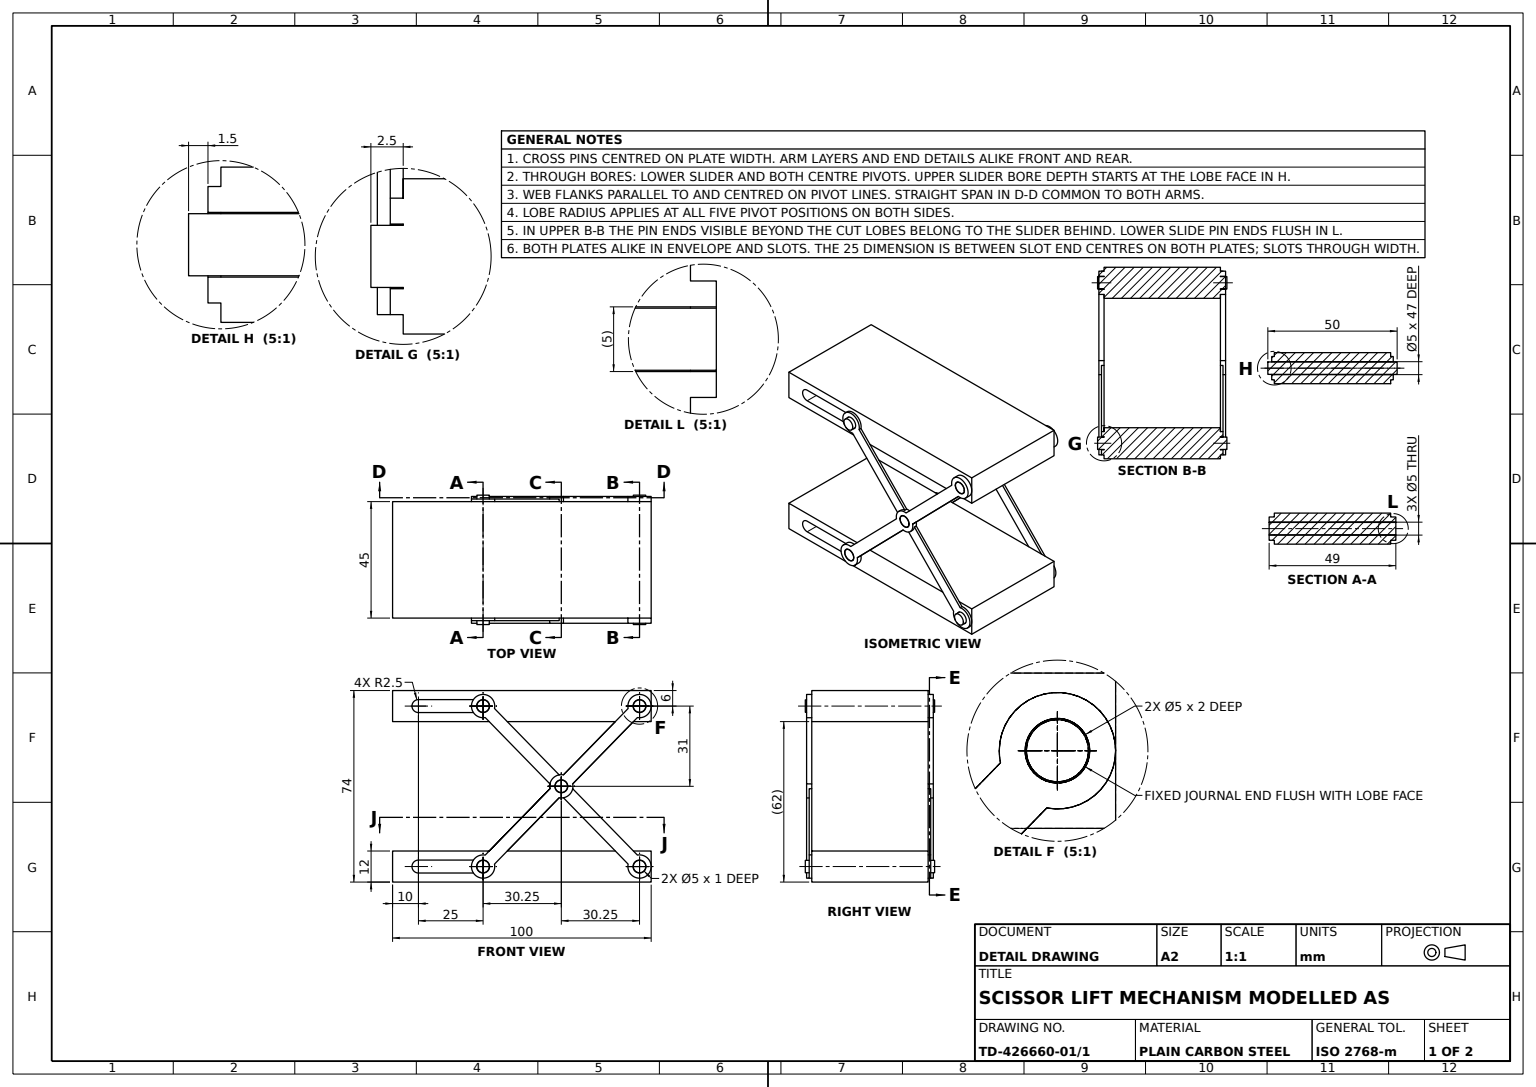
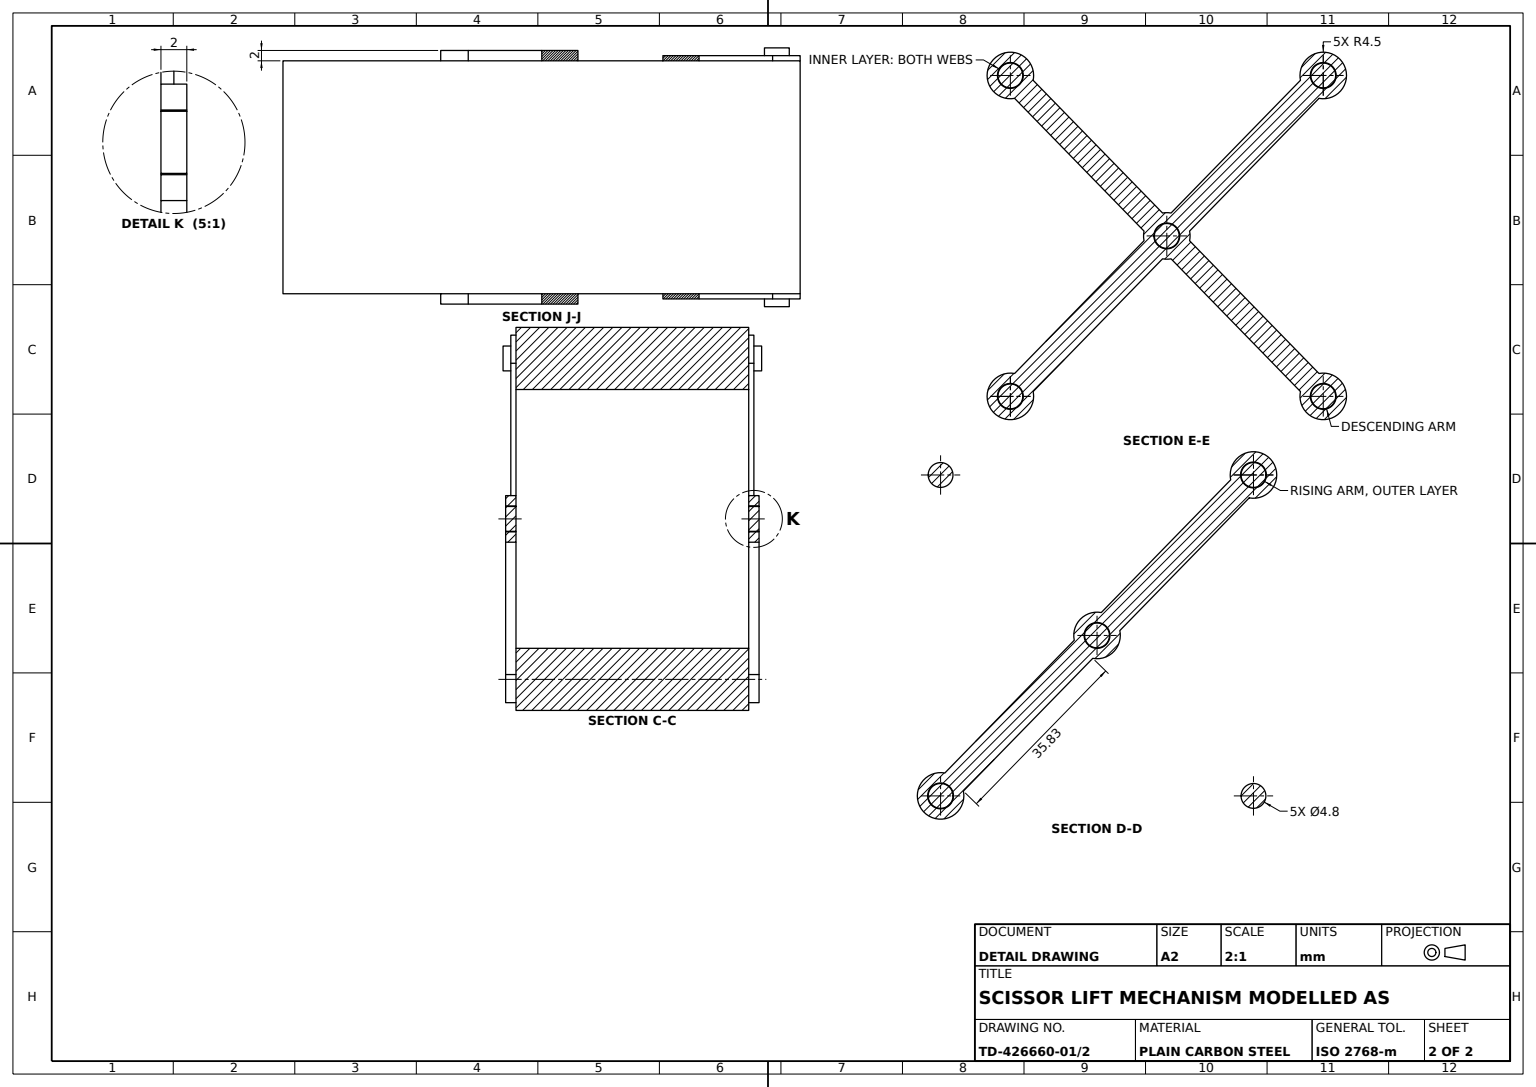
solid
v1 (-17.4,68,-25)
v2 (-12.6,68,-25)
e1 v1 v2 CIRCLE(AX(P(-15,68,-25),D(0,0,-1),D(-1,0,0)),2.4)
e2 v2 v1 CIRCLE(AX(P(-15,68,-25),D(0,0,-1),D(-1,0,0)),2.4)
face PLANE(AX(P(-15,68,-25),D(0,0,-1),D(-1,0,0))) [e1 e2]
v3 (-12.6,68,25)
e3 v3 v2 LINE
v4 (-17.4,68,25)
e4 v4 v3 CIRCLE(AX(P(-15,68,25),D(0,0,1),D(1,0,0)),2.4)
e5 v4 v1 LINE
face CYL(AX(P(-15,68,25),D(0,0,-1),D(-1,0,0)),2.4) [-e3 -e4 e5 -e2]
e6 v3 v4 CIRCLE(AX(P(-15,68,25),D(0,0,1),D(1,0,0)),2.4)
face PLANE(AX(P(-15,68,25),D(0,0,1),D(1,0,0))) [e4 e6]
face CYL(AX(P(-15,68,25),D(0,0,-1),D(-1,0,0)),2.4) [-e5 -e6 e3 -e1]
solid
v5 (17.65,37,22.5)
v6 (12.85,37,22.5)
e7 v5 v6 CIRCLE(AX(P(15.25,37,22.5),D(0,0,1),D(1,0,0)),2.4)
e8 v6 v5 CIRCLE(AX(P(15.25,37,22.5),D(0,0,1),D(1,0,0)),2.4)
face PLANE(AX(P(15.25,37,22.5),D(0,0,1),D(1,0,0))) rev [-e7 -e8]
v7 (17.65,37,24.5)
v8 (12.85,37,24.5)
e9 v7 v8 CIRCLE(AX(P(15.25,37,24.5),D(0,0,1),D(1,0,0)),2.4)
e10 v8 v7 CIRCLE(AX(P(15.25,37,24.5),D(0,0,1),D(1,0,0)),2.4)
face PLANE(AX(P(15.25,37,24.5),D(0,0,1),D(1,0,0))) [e9 e10]
e11 v5 v7 LINE
e12 v6 v8 LINE
face CYL(AX(P(15.25,37,22.5),D(0,0,1),D(1,0,0)),2.4) [-e9 -e11 e7 e12]
face CYL(AX(P(15.25,37,22.5),D(0,0,1),D(1,0,0)),2.4) [e11 -e10 -e12 e8]
solid
v9 (12.85,37,-22.5)
v10 (12.85,37,-24.5)
e13 v9 v10 LINE
v11 (17.65,37,-24.5)
e14 v11 v10 CIRCLE(AX(P(15.25,37,-24.5),D(0,0,-1),D(-1,0,0)),2.4)
v12 (17.65,37,-22.5)
e15 v12 v11 LINE
e16 v12 v9 CIRCLE(AX(P(15.25,37,-22.5),D(0,0,-1),D(-1,0,0)),2.4)
face CYL(AX(P(15.25,37,-22.5),D(0,0,-1),D(-1,0,0)),2.4) [e13 -e14 -e15 e16]
e17 v10 v11 CIRCLE(AX(P(15.25,37,-24.5),D(0,0,-1),D(-1,0,0)),2.4)
face PLANE(AX(P(15.25,37,-24.5),D(0,0,-1),D(-1,0,0))) [e17 e14]
e18 v9 v12 CIRCLE(AX(P(15.25,37,-22.5),D(0,0,-1),D(-1,0,0)),2.4)
face PLANE(AX(P(15.25,37,-22.5),D(0,0,-1),D(-1,0,0))) rev [-e18 -e16]
face CYL(AX(P(15.25,37,-22.5),D(0,0,-1),D(-1,0,0)),2.4) [e15 -e17 -e13 e18]
solid
v13 (-12.6,6,-24.5)
v14 (-12.6,6,24.5)
e19 v13 v14 LINE
v15 (-17.4,6,24.5)
e20 v15 v14 CIRCLE(AX(P(-15,6,24.5),D(0,0,1),D(1,0,0)),2.4)
v16 (-17.4,6,-24.5)
e21 v16 v15 LINE
e22 v16 v13 CIRCLE(AX(P(-15,6,-24.5),D(0,0,1),D(1,0,0)),2.4)
face CYL(AX(P(-15,6,-24.5),D(0,0,1),D(1,0,0)),2.4) [e19 -e20 -e21 e22]
e23 v14 v15 CIRCLE(AX(P(-15,6,24.5),D(0,0,1),D(1,0,0)),2.4)
face PLANE(AX(P(-15,6,24.5),D(0,0,1),D(1,0,0))) [e23 e20]
e24 v13 v16 CIRCLE(AX(P(-15,6,-24.5),D(0,0,1),D(1,0,0)),2.4)
face PLANE(AX(P(-15,6,-24.5),D(0,0,1),D(1,0,0))) rev [-e22 -e24]
face CYL(AX(P(-15,6,-24.5),D(0,0,1),D(1,0,0)),2.4) [e21 -e23 -e19 e24]
solid
v17 (12.75,37,24.5)
v18 (17.75,37,24.5)
e25 v17 v18 CIRCLE(AX(P(15.25,37,24.5),D(0,0,1),D(1,0,0)),2.5)
v19 (17.75,37,22.5)
e26 v18 v19 LINE
v20 (12.75,37,22.5)
e27 v20 v19 CIRCLE(AX(P(15.25,37,22.5),D(0,0,1),D(1,0,0)),2.5)
e28 v17 v20 LINE
face CYL(AX(P(15.25,37,23.5),D(0,0,-1),D(-1,0,0)),2.5) rev [e25 e26 -e27 -e28]
v21 (47.9,68,-22.5)
v22 (43.1,68,-22.5)
e29 v21 v22 CIRCLE(AX(P(45.5,68,-22.5),D(0,0,-1),D(1,0,0)),2.4)
v23 (43.1,68,-24.5)
e30 v23 v22 LINE
v24 (47.9,68,-24.5)
e31 v24 v23 CIRCLE(AX(P(45.5,68,-24.5),D(0,0,-1),D(-1,0,0)),2.4)
e32 v24 v21 LINE
face CYL(AX(P(45.5,68,-24.5),D(0,0,1),D(1,0,0)),2.4) [e29 -e30 -e31 e32]
v25 (-40,8.5,22.5)
v26 (-40,3.5,22.5)
e33 v25 v26 CIRCLE(AX(P(-40,6,22.5),D(0,0,1),D(1,0,0)),2.5)
v27 (-40,3.5,-22.5)
e34 v27 v26 LINE
v28 (-40,8.5,-22.5)
e35 v28 v27 CIRCLE(AX(P(-40,6,-22.5),D(0,0,1),D(1,0,0)),2.5)
e36 v28 v25 LINE
face CYL(AX(P(-40,6,-177.5),D(0,0,1),D(1,0,0)),2.5) rev [e33 -e34 -e35 e36]
v29 (50,68,-22.5)
v30 (44.67612,63.576063,-22.5)
e37 v29 v30 CIRCLE(AX(P(45.5,68,-22.5),D(0,0,-1),D(-1,0,0)),4.5)
v31 (44.67612,63.576063,-24.5)
e38 v31 v30 LINE
v32 (50,68,-24.5)
e39 v32 v31 CIRCLE(AX(P(45.5,68,-24.5),D(0,0,-1),D(-1,0,0)),4.5)
e40 v32 v29 LINE
face CYL(AX(P(45.5,68,-24.5),D(0,0,1),D(1,0,0)),4.5) [e37 -e38 -e39 e40]
v33 (43,6,23.5)
v34 (43,6,22.5)
e41 v33 v34 LINE
v35 (48,6,22.5)
e42 v35 v34 CIRCLE(AX(P(45.5,6,22.5),D(0,0,1),D(1,0,0)),2.5)
v36 (48,6,23.5)
e43 v36 v35 LINE
e44 v36 v33 CIRCLE(AX(P(45.5,6,23.5),D(0,0,1),D(1,0,0)),2.5)
face CYL(AX(P(45.5,6,23.5),D(0,0,-1),D(-1,0,0)),2.5) rev [e41 -e42 -e43 e44]
v37 (-12.638188,12,-22.5)
v38 (10.847563,36.068042,-22.5)
e45 v37 v38 LINE
v39 (10.847563,36.068042,-24.5)
e46 v39 v38 LINE
v40 (-14.17612,10.423937,-24.5)
e47 v40 v39 LINE
v41 (-14.17612,10.423937,-22.5)
e48 v40 v41 LINE
e49 v41 v37 LINE
face PLANE(AX(P(10.847563,36.068042,-24.5),D(0.715711578,-0.698395975,0),D(0.698395975,0.715711578,0))) rev [e45 -e46 -e47 e48 e49]
v42 (16.07388,32.576063,-22.5)
v43 (14.42612,32.576063,-22.5)
e50 v42 v43 CIRCLE(AX(P(15.25,37,-22.5),D(0,0,-1),D(-1,0,0)),4.5)
v44 (14.42612,32.576063,-24.5)
e51 v44 v43 LINE
v45 (19.75,37,-24.5)
e52 v45 v44 CIRCLE(AX(P(15.25,37,-24.5),D(0,0,-1),D(-1,0,0)),4.5)
v46 (19.75,37,-22.5)
e53 v45 v46 LINE
v47 (19.652437,36.068042,-22.5)
e54 v46 v47 CIRCLE(AX(P(15.25,37,-22.5),D(0,0,-1),D(-1,0,0)),4.5)
v48 (19.652437,36.068042,-23.5)
e55 v48 v47 LINE
v49 (16.07388,32.576063,-23.5)
e56 v49 v48 CIRCLE(AX(P(15.25,37,-23.5),D(0,0,1),D(-1,0,0)),4.5)
e57 v49 v42 LINE
face CYL(AX(P(15.25,37,-23.5),D(0,0,1),D(1,0,0)),4.5) [e50 -e51 -e52 e53 e54 -e55 -e56 e57]
v50 (-19.5,6,-24.5)
e58 v50 v40 CIRCLE(AX(P(-15,6,-24.5),D(0,0,-1),D(-1,0,0)),4.5)
v51 (-19.5,6,-22.5)
e59 v50 v51 LINE
v52 (-18.741657,8.5,-22.5)
e60 v51 v52 CIRCLE(AX(P(-15,6,-22.5),D(0,0,-1),D(-1,0,0)),4.5)
e61 v52 v41 CIRCLE(AX(P(-15,6,-22.5),D(0,0,-1),D(-1,0,0)),4.5)
face CYL(AX(P(-15,6,-24.5),D(0,0,1),D(1,0,0)),4.5) [-e58 e59 e60 e61 -e48]
v53 (41,6,-23.5)
v54 (41.097563,6.931958,-23.5)
e62 v53 v54 CIRCLE(AX(P(45.5,6,-23.5),D(0,0,-1),D(-1,0,0)),4.5)
v55 (41,6,-22.5)
e63 v53 v55 LINE
v56 (41.097563,6.931958,-22.5)
e64 v55 v56 CIRCLE(AX(P(45.5,6,-22.5),D(0,0,-1),D(-1,0,0)),4.5)
e65 v54 v56 LINE
face CYL(AX(P(45.5,6,-23.5),D(0,0,1),D(1,0,0)),4.5) [-e62 e63 e64 -e65]
v57 (41,6,23.5)
v58 (41,6,22.5)
e66 v57 v58 LINE
v59 (41.097563,6.931958,23.5)
e67 v59 v57 CIRCLE(AX(P(45.5,6,23.5),D(0,0,1),D(1,0,0)),4.5)
v60 (41.097563,6.931958,22.5)
e68 v59 v60 LINE
e69 v60 v58 CIRCLE(AX(P(45.5,6,22.5),D(0,0,1),D(1,0,0)),4.5)
face CYL(AX(P(45.5,6,23.5),D(0,0,-1),D(-1,0,0)),4.5) [-e66 -e67 e68 e69]
v61 (-5.652134,12,-22.5)
v62 (-10.597563,6.931958,-22.5)
e70 v61 v62 LINE
v63 (36.152134,12,-22.5)
e71 v63 v61 LINE
e72 v56 v63 LINE
v64 (50,6,-22.5)
e73 v64 v55 CIRCLE(AX(P(45.5,6,-22.5),D(0,0,-1),D(-1,0,0)),4.5)
v65 (50,0,-22.5)
e74 v64 v65 LINE
v66 (-50,0,-22.5)
e75 v65 v66 LINE
v67 (-50,12,-22.5)
e76 v67 v66 LINE
e77 v37 v67 LINE
e78 v52 v28 LINE
v68 (-18.741657,3.5,-22.5)
e79 v27 v68 LINE
v69 (-10.5,6,-22.5)
e80 v69 v68 CIRCLE(AX(P(-15,6,-22.5),D(0,0,-1),D(-1,0,0)),4.5)
e81 v62 v69 CIRCLE(AX(P(-15,6,-22.5),D(0,0,-1),D(-1,0,0)),4.5)
face PLANE(AX(P(-50,12,-22.5),D(0,0,1),D(1,0,0))) rev [-e70 -e71 -e72 -e64 -e73 e74 e75 -e76 -e77 -e49 -e61 e78 e35 e79 -e80 -e81]
v70 (-15,3.5,-22.5)
v71 (-15,3.5,22.5)
e82 v70 v71 LINE
e83 v68 v70 LINE
v72 (-18.741657,3.5,22.5)
e84 v26 v72 LINE
e85 v71 v72 LINE
face PLANE(AX(P(-15,3.5,-177.5),D(0,-1,0),D(1,0,0))) rev [-e82 -e83 -e79 e34 e84 -e85]
v73 (14.42612,41.423937,23.5)
v74 (14.42612,41.423937,22.5)
e86 v73 v74 LINE
v75 (10.847563,37.931958,23.5)
e87 v75 v73 CIRCLE(AX(P(15.25,37,23.5),D(0,0,-1),D(1,0,0)),4.5)
v76 (10.847563,37.931958,22.5)
e88 v75 v76 LINE
v77 (10.75,37,22.5)
e89 v76 v77 CIRCLE(AX(P(15.25,37,22.5),D(0,0,1),D(1,0,0)),4.5)
v78 (10.75,37,24.5)
e90 v78 v77 LINE
v79 (16.07388,41.423937,24.5)
e91 v79 v78 CIRCLE(AX(P(15.25,37,24.5),D(0,0,1),D(1,0,0)),4.5)
v80 (16.07388,41.423937,22.5)
e92 v79 v80 LINE
e93 v80 v74 CIRCLE(AX(P(15.25,37,22.5),D(0,0,1),D(1,0,0)),4.5)
face CYL(AX(P(15.25,37,23.5),D(0,0,-1),D(-1,0,0)),4.5) [-e86 -e87 e88 e89 -e90 -e91 e92 e93]
v81 (47.9,6,22.5)
v82 (43.1,6,22.5)
e94 v81 v82 CIRCLE(AX(P(45.5,6,22.5),D(0,0,1),D(-1,0,0)),2.4)
v83 (43.1,6,25)
e95 v83 v82 LINE
v84 (47.9,6,25)
e96 v84 v83 CIRCLE(AX(P(45.5,6,25),D(0,0,1),D(1,0,0)),2.4)
e97 v84 v81 LINE
face CYL(AX(P(45.5,6,25),D(0,0,-1),D(-1,0,0)),2.4) [e94 -e95 -e96 e97]
v85 (16.07388,32.576063,23.5)
e98 v85 v59 LINE
v86 (16.07388,32.576063,22.5)
e99 v85 v86 LINE
v87 (36.152134,12,22.5)
e100 v86 v87 LINE
e101 v87 v60 LINE
face PLANE(AX(P(16.07388,32.576063,23.5),D(0.715711578,0.698395975,0),D(-0.698395975,0.715711578,0))) rev [-e68 -e98 e99 e100 e101]
v88 (10.847563,36.068042,22.5)
e102 v77 v88 CIRCLE(AX(P(15.25,37,22.5),D(0,0,1),D(1,0,0)),4.5)
v89 (10.847563,36.068042,24.5)
e103 v89 v88 LINE
e104 v78 v89 CIRCLE(AX(P(15.25,37,24.5),D(0,0,1),D(1,0,0)),4.5)
face CYL(AX(P(15.25,37,23.5),D(0,0,-1),D(-1,0,0)),4.5) [e90 e102 -e103 -e104]
e105 v82 v81 CIRCLE(AX(P(45.5,6,22.5),D(0,0,1),D(-1,0,0)),2.4)
e106 v83 v84 CIRCLE(AX(P(45.5,6,25),D(0,0,1),D(1,0,0)),2.4)
face CYL(AX(P(45.5,6,25),D(0,0,-1),D(-1,0,0)),2.4) [e95 e105 -e97 -e106]
v90 (41,68,-22.5)
e107 v90 v29 CIRCLE(AX(P(45.5,68,-22.5),D(0,0,-1),D(-1,0,0)),4.5)
v91 (41,68,-24.5)
e108 v91 v32 CIRCLE(AX(P(45.5,68,-24.5),D(0,0,-1),D(-1,0,0)),4.5)
e109 v91 v90 LINE
face CYL(AX(P(45.5,68,-24.5),D(0,0,1),D(1,0,0)),4.5) [e107 -e40 -e108 e109]
v92 (47.9,68,24.5)
v93 (47.9,68,22.5)
e110 v92 v93 LINE
v94 (43.1,68,24.5)
e111 v94 v92 CIRCLE(AX(P(45.5,68,24.5),D(0,0,1),D(1,0,0)),2.4)
v95 (43.1,68,22.5)
e112 v94 v95 LINE
e113 v95 v93 CIRCLE(AX(P(45.5,68,22.5),D(0,0,1),D(-1,0,0)),2.4)
face CYL(AX(P(45.5,68,24.5),D(0,0,-1),D(-1,0,0)),2.4) [-e110 -e111 e112 e113]
v96 (-50,62,-22.5)
v97 (-50,62,22.5)
e114 v96 v97 LINE
v98 (-50,74,22.5)
e115 v98 v97 LINE
v99 (-50,74,-22.5)
e116 v99 v98 LINE
e117 v99 v96 LINE
face PLANE(AX(P(-50,74,-22.5),D(1,0,0),D(0,0,-1))) rev [e114 -e115 -e116 e117]
v100 (19.652437,37.931958,-24.5)
e118 v31 v100 LINE
v101 (43.138188,62,-22.5)
e119 v30 v101 LINE
v102 (19.652437,37.931958,-22.5)
e120 v101 v102 LINE
e121 v100 v102 LINE
face PLANE(AX(P(44.67612,63.576063,-24.5),D(-0.715711578,0.698395975,0),D(-0.698395975,-0.715711578,0))) rev [-e118 e38 e119 e120 -e121]
v103 (50,62,-22.5)
e122 v29 v103 LINE
v104 (50,74,-22.5)
e123 v104 v29 LINE
v105 (50,74,22.5)
e124 v105 v104 LINE
v106 (50,68,22.5)
e125 v105 v106 LINE
v107 (50,62,22.5)
e126 v106 v107 LINE
e127 v107 v103 LINE
face PLANE(AX(P(50,74,-22.5),D(-1,0,0),D(0,0,1))) rev [-e122 -e123 -e124 e125 e126 e127]
v108 (14.42612,41.423937,-23.5)
v109 (14.42612,41.423937,-22.5)
e128 v108 v109 LINE
v110 (-10.597563,67.068042,-23.5)
e129 v110 v108 LINE
v111 (-10.597563,67.068042,-22.5)
e130 v110 v111 LINE
v112 (-5.652134,62,-22.5)
e131 v111 v112 LINE
e132 v112 v109 LINE
face PLANE(AX(P(14.42612,41.423937,-23.5),D(-0.715711578,-0.698395975,0),D(0.698395975,-0.715711578,0))) rev [-e128 -e129 e130 e131 e132]
e133 v68 v51 CIRCLE(AX(P(-15,6,-22.5),D(0,0,-1),D(-1,0,0)),4.5)
v113 (-10.5,6,-24.5)
e134 v113 v50 CIRCLE(AX(P(-15,6,-24.5),D(0,0,-1),D(-1,0,0)),4.5)
e135 v113 v69 LINE
face CYL(AX(P(-15,6,-24.5),D(0,0,1),D(1,0,0)),4.5) [e80 e133 -e59 -e134 e135]
v114 (50,12,22.5)
v115 (50,12,-22.5)
e136 v114 v115 LINE
v116 (43.138188,12,-22.5)
e137 v115 v116 LINE
e138 v116 v63 LINE
e139 v61 v37 LINE
v117 (-50,12,22.5)
e140 v67 v117 LINE
v118 (-12.638188,12,22.5)
e141 v117 v118 LINE
v119 (-5.652134,12,22.5)
e142 v118 v119 LINE
e143 v119 v87 LINE
v120 (43.138188,12,22.5)
e144 v87 v120 LINE
e145 v120 v114 LINE
face PLANE(AX(P(0,12,0),D(0,1,0),D(0,0,1))) [e136 e137 e138 e71 e139 e77 e140 e141 e142 e143 e144 e145]
e146 v22 v21 CIRCLE(AX(P(45.5,68,-22.5),D(0,0,-1),D(1,0,0)),2.4)
e147 v23 v24 CIRCLE(AX(P(45.5,68,-24.5),D(0,0,-1),D(-1,0,0)),2.4)
face CYL(AX(P(45.5,68,-24.5),D(0,0,1),D(1,0,0)),2.4) [e146 -e32 -e147 e30]
v121 (10.847563,37.931958,-23.5)
v122 (-14.17612,63.576063,-23.5)
e148 v121 v122 LINE
v123 (10.847563,37.931958,-22.5)
e149 v121 v123 LINE
v124 (-12.638188,62,-22.5)
e150 v123 v124 LINE
v125 (-14.17612,63.576063,-22.5)
e151 v124 v125 LINE
e152 v122 v125 LINE
face PLANE(AX(P(10.847563,37.931958,-23.5),D(0.715711578,0.698395975,0),D(-0.698395975,0.715711578,0))) rev [-e148 e149 e150 e151 -e152]
v126 (-15,8.5,-22.5)
v127 (-15,8.5,22.5)
e153 v126 v127 LINE
v128 (-18.741657,8.5,22.5)
e154 v127 v128 LINE
e155 v128 v25 LINE
e156 v126 v52 LINE
face PLANE(AX(P(-15,8.5,-177.5),D(0,1,0),D(0,0,1))) rev [e153 e154 e155 -e36 -e78 -e156]
v129 (41,68,24.5)
v130 (41,68,22.5)
e157 v129 v130 LINE
v131 (50,68,24.5)
e158 v131 v129 CIRCLE(AX(P(45.5,68,24.5),D(0,0,1),D(1,0,0)),4.5)
e159 v131 v106 LINE
e160 v106 v130 CIRCLE(AX(P(45.5,68,22.5),D(0,0,1),D(1,0,0)),4.5)
face CYL(AX(P(45.5,68,24.5),D(0,0,-1),D(-1,0,0)),4.5) [-e157 -e158 e159 e160]
v132 (44.67612,10.423937,22.5)
e161 v132 v120 LINE
v133 (50,6,22.5)
e162 v133 v132 CIRCLE(AX(P(45.5,6,22.5),D(0,0,1),D(1,0,0)),4.5)
e163 v114 v133 LINE
face PLANE(AX(P(-50,12,22.5),D(0,0,-1),D(-1,0,0))) rev [-e145 -e161 -e162 -e163]
v134 (50,6,23.5)
e164 v134 v133 LINE
e165 v57 v134 CIRCLE(AX(P(45.5,6,23.5),D(0,0,1),D(1,0,0)),4.5)
e166 v58 v133 CIRCLE(AX(P(45.5,6,22.5),D(0,0,1),D(1,0,0)),4.5)
face CYL(AX(P(45.5,6,23.5),D(0,0,-1),D(-1,0,0)),4.5) [-e164 -e165 e66 e166]
e167 v92 v94 CIRCLE(AX(P(45.5,68,24.5),D(0,0,1),D(1,0,0)),2.4)
e168 v93 v95 CIRCLE(AX(P(45.5,68,22.5),D(0,0,1),D(-1,0,0)),2.4)
face CYL(AX(P(45.5,68,24.5),D(0,0,-1),D(-1,0,0)),2.4) [-e112 -e167 e110 e168]
v135 (-10.5,68,-22.5)
e169 v135 v111 CIRCLE(AX(P(-15,68,-22.5),D(0,0,-1),D(-1,0,0)),4.5)
v136 (-18.741657,70.5,-22.5)
e170 v136 v135 CIRCLE(AX(P(-15,68,-22.5),D(0,0,-1),D(-1,0,0)),4.5)
v137 (-40,70.5,-22.5)
e171 v136 v137 LINE
v138 (-40,65.5,-22.5)
e172 v137 v138 CIRCLE(AX(P(-40,68,-22.5),D(0,0,1),D(1,0,0)),2.5)
v139 (-18.741657,65.5,-22.5)
e173 v138 v139 LINE
e174 v125 v139 CIRCLE(AX(P(-15,68,-22.5),D(0,0,-1),D(-1,0,0)),4.5)
e175 v124 v96 LINE
e176 v104 v99 LINE
v140 (41.097563,67.068042,-22.5)
e177 v140 v90 CIRCLE(AX(P(45.5,68,-22.5),D(0,0,-1),D(-1,0,0)),4.5)
v141 (36.152134,62,-22.5)
e178 v141 v140 LINE
e179 v141 v112 LINE
face PLANE(AX(P(-50,74,-22.5),D(0,0,1),D(1,0,0))) rev [-e169 -e170 e171 e172 e173 -e174 -e151 e175 -e117 -e176 e123 -e107 -e177 -e178 e179 -e131]
v142 (44.67612,10.423937,-23.5)
e180 v48 v142 LINE
e181 v47 v116 LINE
v143 (44.67612,10.423937,-22.5)
e182 v116 v143 LINE
e183 v142 v143 LINE
face PLANE(AX(P(44.67612,10.423937,-23.5),D(-0.715711578,-0.698395975,0),D(0.698395975,-0.715711578,0))) rev [-e180 e55 e181 e182 -e183]
v144 (48,68,-22.5)
v145 (43,68,-22.5)
e184 v144 v145 CIRCLE(AX(P(45.5,68,-22.5),D(0,0,-1),D(-1,0,0)),2.5)
e185 v145 v144 CIRCLE(AX(P(45.5,68,-22.5),D(0,0,-1),D(-1,0,0)),2.5)
face PLANE(AX(P(-50,74,-22.5),D(0,0,1),D(1,0,0))) rev [e184 e185] [-e29 -e146]
v146 (47.9,6,-25)
v147 (47.9,6,-22.5)
e186 v146 v147 LINE
v148 (43.1,6,-22.5)
e187 v147 v148 CIRCLE(AX(P(45.5,6,-22.5),D(0,0,-1),D(1,0,0)),2.4)
v149 (43.1,6,-25)
e188 v149 v148 LINE
e189 v146 v149 CIRCLE(AX(P(45.5,6,-25),D(0,0,-1),D(-1,0,0)),2.4)
face CYL(AX(P(45.5,6,-25),D(0,0,1),D(1,0,0)),2.4) [e186 e187 -e188 -e189]
v150 (48,6,-23.5)
v151 (48,6,-22.5)
e190 v150 v151 LINE
v152 (43,6,-23.5)
e191 v150 v152 CIRCLE(AX(P(45.5,6,-23.5),D(0,0,-1),D(-1,0,0)),2.5)
v153 (43,6,-22.5)
e192 v152 v153 LINE
e193 v151 v153 CIRCLE(AX(P(45.5,6,-22.5),D(0,0,-1),D(-1,0,0)),2.5)
face CYL(AX(P(45.5,6,-23.5),D(0,0,1),D(1,0,0)),2.5) rev [-e190 e191 e192 -e193]
e194 v98 v105 LINE
face PLANE(AX(P(0,74,0),D(0,1,0),D(0,0,1))) [e194 e124 e176 e116]
v154 (43.138188,62,22.5)
v155 (44.67612,63.576063,22.5)
e195 v154 v155 LINE
v156 (44.67612,63.576063,24.5)
e196 v156 v155 LINE
v157 (19.652437,37.931958,24.5)
e197 v157 v156 LINE
v158 (19.652437,37.931958,22.5)
e198 v157 v158 LINE
e199 v158 v154 LINE
face PLANE(AX(P(19.652437,37.931958,24.5),D(-0.715711578,0.698395975,0),D(-0.698395975,-0.715711578,0))) rev [e195 -e196 -e197 e198 e199]
v159 (-10.5,68,-23.5)
e200 v159 v110 CIRCLE(AX(P(-15,68,-23.5),D(0,0,-1),D(-1,0,0)),4.5)
e201 v159 v135 LINE
face CYL(AX(P(-15,68,-23.5),D(0,0,1),D(1,0,0)),4.5) [-e130 -e200 e201 e169]
v160 (14.42612,32.576063,24.5)
v161 (14.42612,32.576063,22.5)
e202 v160 v161 LINE
v162 (-10.597563,6.931958,24.5)
e203 v162 v160 LINE
v163 (-10.597563,6.931958,22.5)
e204 v162 v163 LINE
e205 v163 v119 LINE
e206 v119 v161 LINE
face PLANE(AX(P(-10.597563,6.931958,24.5),D(-0.715711578,0.698395975,0),D(-0.698395975,-0.715711578,0))) rev [-e202 -e203 e204 e205 e206]
v164 (-15,65.5,-22.5)
v165 (-15,65.5,22.5)
e207 v164 v165 LINE
e208 v139 v164 LINE
v166 (-40,65.5,22.5)
e209 v138 v166 LINE
v167 (-18.741657,65.5,22.5)
e210 v166 v167 LINE
e211 v167 v165 LINE
face PLANE(AX(P(-15,65.5,-27.5),D(0,-1,0),D(1,0,0))) rev [-e207 -e208 -e173 e209 e210 e211]
v168 (-19.5,6,22.5)
e212 v168 v72 CIRCLE(AX(P(-15,6,22.5),D(0,0,1),D(1,0,0)),4.5)
v169 (-10.5,6,22.5)
e213 v72 v169 CIRCLE(AX(P(-15,6,22.5),D(0,0,1),D(1,0,0)),4.5)
v170 (-10.5,6,24.5)
e214 v170 v169 LINE
v171 (-19.5,6,24.5)
e215 v171 v170 CIRCLE(AX(P(-15,6,24.5),D(0,0,1),D(1,0,0)),4.5)
e216 v171 v168 LINE
face CYL(AX(P(-15,6,24.5),D(0,0,-1),D(-1,0,0)),4.5) [e212 e213 -e214 -e215 e216]
v172 (43,68,24.5)
v173 (48,68,24.5)
e217 v172 v173 CIRCLE(AX(P(45.5,68,24.5),D(0,0,1),D(1,0,0)),2.5)
v174 (48,68,22.5)
e218 v173 v174 LINE
v175 (43,68,22.5)
e219 v175 v174 CIRCLE(AX(P(45.5,68,22.5),D(0,0,1),D(1,0,0)),2.5)
e220 v172 v175 LINE
face CYL(AX(P(45.5,68,24.5),D(0,0,-1),D(-1,0,0)),2.5) rev [e217 e218 -e219 -e220]
v176 (-14.17612,63.576063,22.5)
e221 v176 v167 CIRCLE(AX(P(-15,68,22.5),D(0,0,-1),D(-1,0,0)),4.5)
v177 (-14.17612,63.576063,23.5)
e222 v177 v176 LINE
v178 (-19.5,68,23.5)
e223 v178 v177 CIRCLE(AX(P(-15,68,23.5),D(0,0,1),D(1,0,0)),4.5)
v179 (-19.5,68,22.5)
e224 v178 v179 LINE
e225 v179 v167 CIRCLE(AX(P(-15,68,22.5),D(0,0,1),D(1,0,0)),4.5)
face CYL(AX(P(-15,68,23.5),D(0,0,-1),D(-1,0,0)),4.5) [-e221 -e222 -e223 e224 e225]
e226 v18 v17 CIRCLE(AX(P(15.25,37,24.5),D(0,0,1),D(1,0,0)),2.5)
e227 v173 v172 CIRCLE(AX(P(45.5,68,24.5),D(0,0,1),D(1,0,0)),2.5)
v180 (-17.5,6,24.5)
v181 (-12.5,6,24.5)
e228 v180 v181 CIRCLE(AX(P(-15,6,24.5),D(0,0,1),D(1,0,0)),2.5)
e229 v181 v180 CIRCLE(AX(P(-15,6,24.5),D(0,0,1),D(1,0,0)),2.5)
v182 (-14.17612,10.423937,24.5)
e230 v89 v182 LINE
e231 v182 v171 CIRCLE(AX(P(-15,6,24.5),D(0,0,1),D(1,0,0)),4.5)
e232 v170 v162 CIRCLE(AX(P(-15,6,24.5),D(0,0,1),D(1,0,0)),4.5)
e233 v160 v157 CIRCLE(AX(P(15.25,37,24.5),D(0,0,1),D(1,0,0)),4.5)
e234 v156 v131 CIRCLE(AX(P(45.5,68,24.5),D(0,0,1),D(1,0,0)),4.5)
v183 (41.097563,67.068042,24.5)
e235 v129 v183 CIRCLE(AX(P(45.5,68,24.5),D(0,0,1),D(1,0,0)),4.5)
e236 v183 v79 LINE
face PLANE(AX(P(-15,6,24.5),D(0,0,1),D(1,0,0))) [-e25 -e226] [-e227 -e217] [-e228 -e229] [e230 e231 e215 e232 e203 e233 e197 e234 e158 e235 e236 e91 e104]
v184 (-18.741657,70.5,22.5)
e237 v184 v179 CIRCLE(AX(P(-15,68,22.5),D(0,0,1),D(1,0,0)),4.5)
v185 (-15,70.5,22.5)
e238 v185 v184 LINE
v186 (-17.5,68,22.5)
e239 v185 v186 CIRCLE(AX(P(-15,68,22.5),D(0,0,1),D(1,0,0)),2.5)
e240 v186 v165 CIRCLE(AX(P(-15,68,22.5),D(0,0,1),D(1,0,0)),2.5)
face PLANE(AX(P(-15,68,22.5),D(0,0,1),D(1,0,0))) rev [-e237 -e238 e239 e240 -e211 -e225]
v187 (-50,0,22.5)
e241 v66 v187 LINE
e242 v117 v187 LINE
face PLANE(AX(P(-50,12,-22.5),D(1,0,0),D(0,0,-1))) rev [e241 -e242 -e140 e76]
v188 (-14.17612,10.423937,22.5)
e243 v182 v188 LINE
e244 v188 v128 CIRCLE(AX(P(-15,6,22.5),D(0,0,1),D(1,0,0)),4.5)
e245 v128 v168 CIRCLE(AX(P(-15,6,22.5),D(0,0,1),D(1,0,0)),4.5)
face CYL(AX(P(-15,6,24.5),D(0,0,-1),D(-1,0,0)),4.5) [-e216 -e231 e243 e244 e245]
v189 (44.67612,10.423937,23.5)
v190 (19.652437,36.068042,23.5)
e246 v189 v190 LINE
e247 v190 v85 CIRCLE(AX(P(15.25,37,23.5),D(0,0,-1),D(1,0,0)),4.5)
e248 v134 v189 CIRCLE(AX(P(45.5,6,23.5),D(0,0,1),D(1,0,0)),4.5)
e249 v33 v36 CIRCLE(AX(P(45.5,6,23.5),D(0,0,1),D(1,0,0)),2.5)
face PLANE(AX(P(-15,68,23.5),D(0,0,1),D(1,0,0))) [e246 e247 e98 e67 e165 e248] [-e249 -e44]
e250 v148 v147 CIRCLE(AX(P(45.5,6,-22.5),D(0,0,-1),D(1,0,0)),2.4)
e251 v153 v151 CIRCLE(AX(P(45.5,6,-22.5),D(0,0,-1),D(-1,0,0)),2.5)
face PLANE(AX(P(-50,12,-22.5),D(0,0,1),D(1,0,0))) rev [-e250 -e187] [e251 e193]
v191 (-17.5,6,-22.5)
e252 v70 v191 CIRCLE(AX(P(-15,6,-22.5),D(0,0,-1),D(-1,0,0)),2.5)
e253 v191 v126 CIRCLE(AX(P(-15,6,-22.5),D(0,0,-1),D(-1,0,0)),2.5)
face PLANE(AX(P(-15,6,-22.5),D(0,0,-1),D(-1,0,0))) rev [-e133 e83 e252 e253 e156 -e60]
v192 (-10.597563,6.931958,-24.5)
e254 v192 v62 LINE
e255 v44 v192 LINE
e256 v43 v61 LINE
face PLANE(AX(P(14.42612,32.576063,-24.5),D(-0.715711578,0.698395975,0),D(-0.698395975,-0.715711578,0))) rev [-e254 -e255 e51 e256 e70]
v193 (-17.5,6,22.5)
e257 v193 v180 LINE
e258 v127 v193 CIRCLE(AX(P(-15,6,22.5),D(0,0,1),D(1,0,0)),2.5)
v194 (-17.5,6,-24.5)
e259 v194 v191 LINE
v195 (-12.5,6,-24.5)
e260 v194 v195 CIRCLE(AX(P(-15,6,-24.5),D(0,0,-1),D(-1,0,0)),2.5)
e261 v195 v181 LINE
face CYL(AX(P(-15,6,-177.5),D(0,0,1),D(1,0,0)),2.5) rev [-e257 -e258 -e153 -e253 -e259 e260 e261 e229]
v196 (-40,70.5,22.5)
e262 v184 v196 LINE
e263 v137 v196 LINE
v197 (-15,70.5,-22.5)
e264 v197 v136 LINE
e265 v197 v185 LINE
face PLANE(AX(P(-15,70.5,-27.5),D(0,1,0),D(-1,0,0))) rev [e238 e262 -e263 -e171 -e264 e265]
v198 (50,0,22.5)
e266 v133 v198 LINE
e267 v198 v65 LINE
e268 v115 v64 LINE
face PLANE(AX(P(50,12,-22.5),D(-1,0,0),D(0,0,1))) rev [-e136 e163 e266 e267 -e74 -e268]
v199 (17.75,37,-24.5)
v200 (17.75,37,-22.5)
e269 v199 v200 LINE
v201 (12.75,37,-24.5)
e270 v199 v201 CIRCLE(AX(P(15.25,37,-24.5),D(0,0,-1),D(-1,0,0)),2.5)
v202 (12.75,37,-22.5)
e271 v201 v202 LINE
e272 v200 v202 CIRCLE(AX(P(15.25,37,-22.5),D(0,0,-1),D(-1,0,0)),2.5)
face CYL(AX(P(15.25,37,-23.5),D(0,0,1),D(1,0,0)),2.5) rev [-e269 e270 e271 -e272]
v203 (-10.5,68,23.5)
e273 v203 v178 CIRCLE(AX(P(-15,68,23.5),D(0,0,1),D(1,0,0)),4.5)
v204 (-10.5,68,22.5)
e274 v203 v204 LINE
e275 v204 v184 CIRCLE(AX(P(-15,68,22.5),D(0,0,1),D(1,0,0)),4.5)
face CYL(AX(P(-15,68,23.5),D(0,0,-1),D(-1,0,0)),4.5) [e237 -e224 -e273 e274 e275]
e276 v174 v175 CIRCLE(AX(P(45.5,68,22.5),D(0,0,1),D(1,0,0)),2.5)
face CYL(AX(P(45.5,68,24.5),D(0,0,-1),D(-1,0,0)),2.5) rev [e227 e220 -e276 -e218]
v205 (41.097563,67.068042,22.5)
v206 (36.152134,62,22.5)
e277 v205 v206 LINE
e278 v206 v80 LINE
e279 v183 v205 LINE
face PLANE(AX(P(16.07388,41.423937,24.5),D(0.715711578,-0.698395975,0),D(0.698395975,0.715711578,0))) rev [e277 e278 -e92 -e236 e279]
e280 v34 v35 CIRCLE(AX(P(45.5,6,22.5),D(0,0,1),D(1,0,0)),2.5)
face CYL(AX(P(45.5,6,23.5),D(0,0,-1),D(-1,0,0)),2.5) rev [e43 -e280 -e41 e249]
e281 v155 v106 CIRCLE(AX(P(45.5,68,22.5),D(0,0,1),D(1,0,0)),4.5)
face CYL(AX(P(45.5,68,24.5),D(0,0,-1),D(-1,0,0)),4.5) [e281 -e159 -e234 e196]
v207 (-5.652134,62,22.5)
e282 v207 v206 LINE
e283 v130 v205 CIRCLE(AX(P(45.5,68,22.5),D(0,0,1),D(1,0,0)),4.5)
v208 (-12.638188,62,22.5)
e284 v97 v208 LINE
e285 v176 v208 LINE
e286 v196 v166 CIRCLE(AX(P(-40,68,22.5),D(0,0,1),D(1,0,0)),2.5)
v209 (-10.597563,67.068042,22.5)
e287 v209 v204 CIRCLE(AX(P(-15,68,22.5),D(0,0,1),D(1,0,0)),4.5)
e288 v209 v207 LINE
face PLANE(AX(P(-50,74,22.5),D(0,0,-1),D(-1,0,0))) rev [e282 -e277 -e283 -e160 -e125 -e194 e115 e284 -e285 e221 -e210 -e286 -e262 -e275 -e287 e288]
v210 (48,68,-24.5)
e289 v210 v144 LINE
v211 (43,68,-24.5)
e290 v211 v145 LINE
e291 v211 v210 CIRCLE(AX(P(45.5,68,-24.5),D(0,0,-1),D(-1,0,0)),2.5)
face CYL(AX(P(45.5,68,-24.5),D(0,0,1),D(1,0,0)),2.5) rev [e289 -e185 -e290 e291]
e292 v193 v71 CIRCLE(AX(P(-15,6,22.5),D(0,0,1),D(1,0,0)),2.5)
face PLANE(AX(P(-15,6,22.5),D(0,0,1),D(1,0,0))) rev [-e212 -e245 -e154 e258 e292 e85]
v212 (-19.5,68,-23.5)
e293 v212 v159 CIRCLE(AX(P(-15,68,-23.5),D(0,0,-1),D(-1,0,0)),4.5)
v213 (-19.5,68,-22.5)
e294 v212 v213 LINE
e295 v213 v136 CIRCLE(AX(P(-15,68,-22.5),D(0,0,-1),D(-1,0,0)),4.5)
face CYL(AX(P(-15,68,-23.5),D(0,0,1),D(1,0,0)),4.5) [-e201 -e293 e294 e295 e170]
e296 v19 v20 CIRCLE(AX(P(15.25,37,22.5),D(0,0,1),D(1,0,0)),2.5)
v214 (19.652437,36.068042,22.5)
e297 v120 v214 LINE
e298 v161 v86 CIRCLE(AX(P(15.25,37,22.5),D(0,0,1),D(1,0,0)),4.5)
e299 v88 v118 LINE
e300 v208 v76 LINE
e301 v208 v207 LINE
e302 v74 v207 LINE
e303 v206 v154 LINE
e304 v214 v158 CIRCLE(AX(P(15.25,37,22.5),D(0,0,1),D(1,0,0)),4.5)
face PLANE(AX(P(-15,68,22.5),D(0,0,1),D(1,0,0))) rev [e296 e27] [-e297 -e144 -e100 -e298 -e206 -e142 -e299 -e102 -e89 -e300 e301 -e302 -e93 -e278 e303 -e199 -e304]
v215 (41.097563,67.068042,-24.5)
e305 v215 v140 LINE
e306 v215 v91 CIRCLE(AX(P(45.5,68,-24.5),D(0,0,-1),D(-1,0,0)),4.5)
face CYL(AX(P(45.5,68,-24.5),D(0,0,1),D(1,0,0)),4.5) [e305 e177 -e109 -e306]
v216 (-10.597563,67.068042,23.5)
e307 v216 v209 LINE
e308 v73 v216 LINE
face PLANE(AX(P(-10.597563,67.068042,23.5),D(-0.715711578,-0.698395975,0),D(0.698395975,-0.715711578,0))) rev [-e288 -e307 -e308 e86 e302]
face PLANE(AX(P(45.5,6,25),D(0,0,1),D(1,0,0))) [e106 e96]
e309 v152 v150 CIRCLE(AX(P(45.5,6,-23.5),D(0,0,-1),D(-1,0,0)),2.5)
face CYL(AX(P(45.5,6,-23.5),D(0,0,1),D(1,0,0)),2.5) rev [e190 -e251 -e192 e309]
e310 v143 v64 CIRCLE(AX(P(45.5,6,-22.5),D(0,0,-1),D(-1,0,0)),4.5)
face PLANE(AX(P(-50,12,-22.5),D(0,0,1),D(1,0,0))) rev [-e310 -e182 -e137 e268]
face CYL(AX(P(-40,68,-27.5),D(0,0,1),D(1,0,0)),2.5) rev [-e209 -e172 e263 e286]
e311 v187 v198 LINE
face PLANE(AX(P(0,0,0),D(0,1,0),D(0,0,1))) rev [-e267 -e311 -e241 -e75]
e312 v100 v45 CIRCLE(AX(P(15.25,37,-24.5),D(0,0,-1),D(-1,0,0)),4.5)
e313 v192 v113 CIRCLE(AX(P(-15,6,-24.5),D(0,0,-1),D(-1,0,0)),4.5)
v217 (16.07388,41.423937,-24.5)
e314 v39 v217 CIRCLE(AX(P(15.25,37,-24.5),D(0,0,-1),D(-1,0,0)),4.5)
e315 v217 v215 LINE
e316 v201 v199 CIRCLE(AX(P(15.25,37,-24.5),D(0,0,-1),D(-1,0,0)),2.5)
e317 v210 v211 CIRCLE(AX(P(45.5,68,-24.5),D(0,0,-1),D(-1,0,0)),2.5)
e318 v195 v194 CIRCLE(AX(P(-15,6,-24.5),D(0,0,-1),D(-1,0,0)),2.5)
face PLANE(AX(P(-15,6,-24.5),D(0,0,-1),D(-1,0,0))) [e108 e39 e118 e312 e52 e255 e313 e134 e58 e47 e314 e315 e306] [-e270 -e316] [-e317 -e291] [-e260 -e318]
v218 (50,6,-23.5)
e319 v218 v64 LINE
e320 v218 v53 CIRCLE(AX(P(45.5,6,-23.5),D(0,0,-1),D(-1,0,0)),4.5)
face CYL(AX(P(45.5,6,-23.5),D(0,0,1),D(1,0,0)),4.5) [e319 e73 -e63 -e320]
e321 v118 v188 LINE
face PLANE(AX(P(-14.17612,10.423937,24.5),D(0.715711578,-0.698395975,0),D(0.698395975,0.715711578,0))) rev [e321 -e243 -e230 e103 e299]
e322 v122 v212 CIRCLE(AX(P(-15,68,-23.5),D(0,0,-1),D(-1,0,0)),4.5)
e323 v139 v213 CIRCLE(AX(P(-15,68,-22.5),D(0,0,-1),D(-1,0,0)),4.5)
face CYL(AX(P(-15,68,-23.5),D(0,0,1),D(1,0,0)),4.5) [-e294 -e322 e152 e174 e323]
e324 v103 v101 LINE
face PLANE(AX(P(-50,74,-22.5),D(0,0,1),D(1,0,0))) rev [e324 -e119 -e37 e122]
e325 v38 v123 CIRCLE(AX(P(15.25,37,-22.5),D(0,0,-1),D(-1,0,0)),4.5)
e326 v108 v121 CIRCLE(AX(P(15.25,37,-23.5),D(0,0,1),D(-1,0,0)),4.5)
v219 (16.07388,41.423937,-22.5)
e327 v109 v219 CIRCLE(AX(P(15.25,37,-22.5),D(0,0,-1),D(-1,0,0)),4.5)
e328 v217 v219 LINE
face CYL(AX(P(15.25,37,-23.5),D(0,0,1),D(1,0,0)),4.5) [-e314 e46 e325 -e149 -e326 e128 e327 -e328]
face CYL(AX(P(45.5,68,-24.5),D(0,0,1),D(1,0,0)),2.5) rev [e290 -e184 -e289 e317]
face CYL(AX(P(15.25,37,23.5),D(0,0,-1),D(-1,0,0)),2.5) rev [e28 -e296 -e26 e226]
v220 (-17.5,68,-23.5)
v221 (-12.5,68,-23.5)
e329 v220 v221 CIRCLE(AX(P(-15,68,-23.5),D(0,0,-1),D(-1,0,0)),2.5)
e330 v221 v220 CIRCLE(AX(P(-15,68,-23.5),D(0,0,-1),D(-1,0,0)),2.5)
face PLANE(AX(P(45.5,6,-23.5),D(0,0,-1),D(-1,0,0))) [-e329 -e330] [e326 e148 e322 e293 e200 e129]
e331 v202 v200 CIRCLE(AX(P(15.25,37,-22.5),D(0,0,-1),D(-1,0,0)),2.5)
face CYL(AX(P(15.25,37,-23.5),D(0,0,1),D(1,0,0)),2.5) rev [e316 e269 -e331 -e271]
face PLANE(AX(P(45.5,68,24.5),D(0,0,1),D(1,0,0))) [e167 e111]
face PLANE(AX(P(-50,12,22.5),D(0,0,-1),D(-1,0,0))) rev [e42 e280] [-e94 -e105]
e332 v154 v107 LINE
face PLANE(AX(P(-50,74,22.5),D(0,0,-1),D(-1,0,0))) rev [-e195 e332 -e126 -e281]
v222 (-17.5,68,-22.5)
e333 v222 v197 CIRCLE(AX(P(-15,68,-22.5),D(0,0,-1),D(-1,0,0)),2.5)
e334 v222 v220 LINE
v223 (-12.5,68,23.5)
e335 v223 v221 LINE
v224 (-17.5,68,23.5)
e336 v223 v224 CIRCLE(AX(P(-15,68,23.5),D(0,0,1),D(1,0,0)),2.5)
e337 v224 v186 LINE
face CYL(AX(P(-15,68,23.5),D(0,0,-1),D(-1,0,0)),2.5) rev [-e265 -e333 e334 e329 -e335 e336 e337 -e239]
e338 v112 v124 LINE
e339 v101 v141 LINE
face PLANE(AX(P(0,62,0),D(0,1,0),D(0,0,1))) rev [-e282 -e301 -e284 -e114 -e175 -e338 -e179 -e339 -e324 -e127 -e332 -e303]
e340 v216 v203 CIRCLE(AX(P(-15,68,23.5),D(0,0,1),D(1,0,0)),4.5)
face CYL(AX(P(-15,68,23.5),D(0,0,-1),D(-1,0,0)),4.5) [e307 e287 -e274 -e340]
e341 v164 v222 CIRCLE(AX(P(-15,68,-22.5),D(0,0,-1),D(-1,0,0)),2.5)
face PLANE(AX(P(45.5,6,-22.5),D(0,0,-1),D(-1,0,0))) rev [-e295 -e323 e208 e341 e333 e264]
e342 v224 v223 CIRCLE(AX(P(-15,68,23.5),D(0,0,1),D(1,0,0)),2.5)
e343 v177 v75 LINE
face PLANE(AX(P(-15,68,23.5),D(0,0,1),D(1,0,0))) [-e336 -e342] [e340 e273 e223 e343 e87 e308]
face CYL(AX(P(-15,6,-24.5),D(0,0,1),D(1,0,0)),4.5) [e254 e81 -e135 -e313]
e344 v149 v146 CIRCLE(AX(P(45.5,6,-25),D(0,0,-1),D(-1,0,0)),2.4)
face PLANE(AX(P(45.5,6,-25),D(0,0,-1),D(-1,0,0))) [e189 e344]
e345 v219 v141 LINE
face PLANE(AX(P(41.097563,67.068042,-24.5),D(0.715711578,-0.698395975,0),D(0.698395975,0.715711578,0))) rev [e328 e345 e178 -e305 -e315]
face CYL(AX(P(45.5,6,-25),D(0,0,1),D(1,0,0)),2.4) [-e344 e188 e250 -e186]
e346 v169 v163 CIRCLE(AX(P(-15,6,22.5),D(0,0,1),D(1,0,0)),4.5)
face CYL(AX(P(-15,6,24.5),D(0,0,-1),D(-1,0,0)),4.5) [-e232 e214 e346 -e204]
e347 v189 v132 LINE
e348 v190 v214 LINE
face PLANE(AX(P(19.652437,36.068042,23.5),D(-0.715711578,-0.698395975,0),D(0.698395975,-0.715711578,0))) rev [-e246 e347 e161 e297 -e348]
e349 v142 v218 CIRCLE(AX(P(45.5,6,-23.5),D(0,0,-1),D(-1,0,0)),4.5)
face CYL(AX(P(45.5,6,-23.5),D(0,0,1),D(1,0,0)),4.5) [e183 e310 -e319 -e349]
face PLANE(AX(P(-50,12,22.5),D(0,0,-1),D(-1,0,0))) rev [-e244 -e321 -e141 e242 e311 -e266 -e166 -e69 -e101 -e143 -e205 -e346 -e213 -e84 -e33 -e155]
face PLANE(AX(P(-50,74,22.5),D(0,0,-1),D(-1,0,0))) rev [-e113 -e168] [e276 e219]
face PLANE(AX(P(-14.17612,63.576063,23.5),D(0.715711578,0.698395975,0),D(-0.698395975,0.715711578,0))) rev [e300 -e88 -e343 e222 e285]
face CYL(AX(P(45.5,68,24.5),D(0,0,-1),D(-1,0,0)),4.5) [-e279 -e235 e157 e283]
face CYL(AX(P(-15,68,23.5),D(0,0,-1),D(-1,0,0)),2.5) rev [e335 e330 -e334 -e341 e207 -e240 -e337 e342]
e350 v63 v42 LINE
e351 v54 v49 LINE
face PLANE(AX(P(41.097563,6.931958,-23.5),D(0.715711578,0.698395975,0),D(-0.698395975,0.715711578,0))) rev [e72 e350 -e57 -e351 e65]
e352 v102 v46 CIRCLE(AX(P(15.25,37,-22.5),D(0,0,-1),D(-1,0,0)),4.5)
face CYL(AX(P(15.25,37,-23.5),D(0,0,1),D(1,0,0)),4.5) [-e312 e121 e352 -e53]
face PLANE(AX(P(45.5,6,-23.5),D(0,0,-1),D(-1,0,0))) [-e309 -e191] [e320 e62 e351 e56 e180 e349]
face CYL(AX(P(15.25,37,23.5),D(0,0,-1),D(-1,0,0)),4.5) [e298 -e99 -e247 e348 e304 -e198 -e233 e202]
face PLANE(AX(P(45.5,68,-24.5),D(0,0,-1),D(-1,0,0))) [e31 e147]
face CYL(AX(P(-15,6,-177.5),D(0,0,1),D(1,0,0)),2.5) rev [e228 -e261 e318 e259 -e252 e82 -e292 e257]
face CYL(AX(P(45.5,6,23.5),D(0,0,-1),D(-1,0,0)),4.5) [-e347 -e248 e164 e162]
face PLANE(AX(P(45.5,6,-22.5),D(0,0,-1),D(-1,0,0))) rev [e331 e272] [-e132 e338 -e150 -e325 -e45 -e139 -e256 -e50 -e350 -e138 -e181 -e54 -e352 -e120 e339 -e345 -e327]
